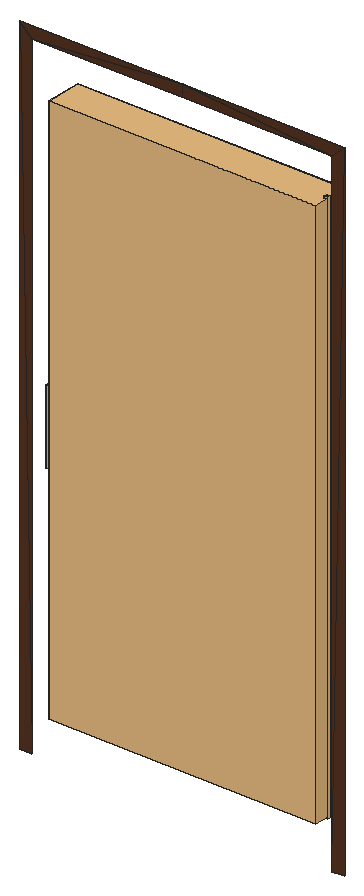
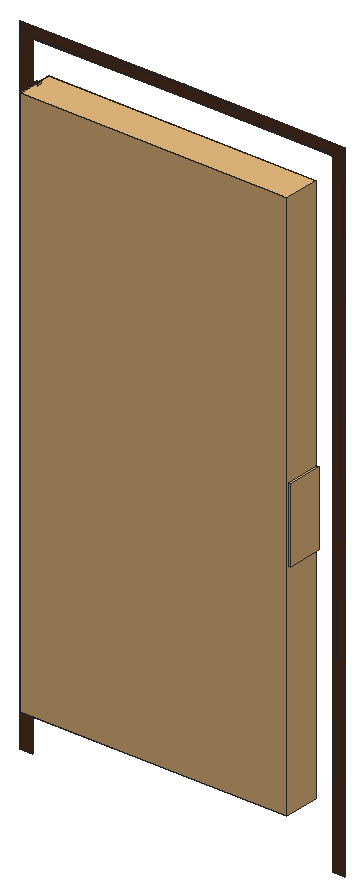
# SketchUp Ruby script. Lengths in inches.
U = 1.inch
M = Sketchup.active_model
def pt(a) = Geom::Point3d.new(a.map { |v| v * U })
def face(e, loops, mat)
  f = e.add_face(loops[0].map { |a| pt(a) })
  loops[1..].each { |l| e.add_face(l.map { |a| pt(a) }).erase! }
  f.material = f.back_material = mat if mat
  f
end
# faces: each face lists its corners as indices into pts; further lists are holes
def faces(e, pts, list, mat = nil) = list.each { |f| face(e, (f[0].is_a?(Array) ? f : [f]).map { |l| l.map { |i| pts[i] } }, mat) }
# xy, xz, yz: faces in a plane at the given z, y or x. An outline is a flat list of corners, or four numbers for a rectangle; further outlines are holes
def ring(l) = l.size == 4 ? [[l[0], l[1]], [l[2], l[1]], [l[2], l[3]], [l[0], l[3]]] : l.each_slice(2).to_a
def flat(e, list, mat, &to3) = list.each { |f| face(e, (f[0].is_a?(Array) ? f : [f]).map { |l| ring(l).map { |u, v| to3.(u, v) } }, mat) }
def xy(e, z, list, mat = nil) = flat(e, list, mat) { |x, y| [x, y, z] }
def xz(e, y, list, mat = nil) = flat(e, list, mat) { |x, z| [x, y, z] }
def yz(e, x, list, mat = nil) = flat(e, list, mat) { |y, z| [x, y, z] }
def lines(e, pts, list) = list.each { |a, b| e.add_line(pt(pts[a]), pt(pts[b])) }
# prism: a flat outline (further loops are holes) pulled along v
def prism(e, loops, v, mat = nil)
  f = face(e, loops, mat); d = Geom::Vector3d.new(v.map { |x| x * U })
  f.pushpull(f.normal.samedirection?(d) ? d.length : -d.length)
end
def box(e, o, s, mat = nil) = prism(e, [[o, [o[0] + s[0], o[1], o[2]], [o[0] + s[0], o[1] + s[1], o[2]], [o[0], o[1] + s[1], o[2]]]], [0, 0, s[2]], mat)
def at(x, y, z, deg = 0) = Geom::Transformation.translation(pt([x, y, z])) * Geom::Transformation.rotation(ORIGIN, Z_AXIS, deg.degrees)
def axes(o, x, y, z) = Geom::Transformation.new([*x, 0, *y, 0, *z, 0, *pt(o).to_a, 1])
def part(name) = M.definitions.add(name)
# library, detail: a bought-in or finely detailed component or shape, given as its bounding box
def library(name, o, s) = part(name).tap { |d| box(d.entities, o, s) }
def detail(e, o, s) = box(e.add_group.entities, o, s)
def put(e, d, t, mat = nil) = e.add_instance(d, t).tap { |i| i.material = mat if mat }
def group(e, t, mat = nil) = e.add_group.tap { |g| g.transformation = t; g.material = mat if mat }.entities
root = M.entities
M.materials.add("Material \#0").color = [86, 53, 35]
M.materials.add("Material \#1").color = [140, 140, 140]
c1 = library("3DGeom~7_Defintion",[455.56,-471.94,-18.85],[5.55,1000,5.48])
c2 = part("3DGeom~8_Defintion")
xz(c2.entities,-471.94,[[458.125,-17.29,459.53,-16.11,457.73,-17.15],[458.125,-17.29,458.54,-17.29,459.53,-16.11],[458.54,-17.29,458.93,-17.15,459.53,-16.11],[457.73,-17.15,459.53,-16.11,457.42,-16.88],[458.93,-17.15,459.25,-16.88,459.53,-16.11],
  [457.42,-16.88,459.53,-16.11,457.21,-16.52],[459.25,-16.88,459.46,-16.52,459.53,-16.11],[457.21,-16.52,459.53,-16.11,457.14,-16.11],[457.14,-16.11,459.53,-16.11,457.21,-15.7],[459.53,-16.11,457.42,-15.34,457.21,-15.7],
  [459.53,-16.11,457.73,-15.07,457.42,-15.34],[459.53,-16.11,458.125,-14.93,457.73,-15.07],[459.53,-16.11,458.54,-14.93,458.125,-14.93],[459.53,-16.11,458.93,-15.07,458.54,-14.93],[459.53,-16.11,459.25,-15.34,458.93,-15.07],
  [459.53,-16.11,459.46,-15.7,459.25,-15.34]],"Material \#1")
xz(c2.entities,-416.39,[[458.125,-17.29,457.73,-17.15,459.53,-16.11],[458.125,-17.29,459.53,-16.11,458.54,-17.29],[458.54,-17.29,459.53,-16.11,458.93,-17.15],[457.73,-17.15,457.42,-16.88,459.53,-16.11],[458.93,-17.15,459.53,-16.11,459.25,-16.88],
  [457.42,-16.88,457.21,-16.52,459.53,-16.11],[459.25,-16.88,459.53,-16.11,459.46,-16.52],[457.21,-16.52,457.14,-16.11,459.53,-16.11],[457.14,-16.11,457.21,-15.7,459.53,-16.11],[459.53,-16.11,457.21,-15.7,457.42,-15.34],
  [459.53,-16.11,457.42,-15.34,457.73,-15.07],[459.53,-16.11,457.73,-15.07,458.125,-14.93],[459.53,-16.11,458.125,-14.93,458.54,-14.93],[459.53,-16.11,458.54,-14.93,458.93,-15.07],[459.53,-16.11,458.93,-15.07,459.25,-15.34],
  [459.53,-16.11,459.25,-15.34,459.46,-15.7]],"Material \#1")
xz(c2.entities,-27.5,[[458.125,-17.29,459.53,-16.11,457.73,-17.15],[458.125,-17.29,458.54,-17.29,459.53,-16.11],[458.54,-17.29,458.93,-17.15,459.53,-16.11],[457.73,-17.15,459.53,-16.11,457.42,-16.88],[458.93,-17.15,459.25,-16.88,459.53,-16.11],
  [457.42,-16.88,459.53,-16.11,457.21,-16.52],[459.25,-16.88,459.46,-16.52,459.53,-16.11],[457.21,-16.52,459.53,-16.11,457.14,-16.11],[457.14,-16.11,459.53,-16.11,457.21,-15.7],[459.53,-16.11,457.42,-15.34,457.21,-15.7],
  [459.53,-16.11,457.73,-15.07,457.42,-15.34],[459.53,-16.11,458.125,-14.93,457.73,-15.07],[459.53,-16.11,458.54,-14.93,458.125,-14.93],[459.53,-16.11,458.93,-15.07,458.54,-14.93],[459.53,-16.11,459.25,-15.34,458.93,-15.07],
  [459.53,-16.11,459.46,-15.7,459.25,-15.34]],"Material \#1")
xz(c2.entities,28.06,[[458.125,-17.29,457.73,-17.15,459.53,-16.11],[458.125,-17.29,459.53,-16.11,458.54,-17.29],[458.54,-17.29,459.53,-16.11,458.93,-17.15],[457.73,-17.15,457.42,-16.88,459.53,-16.11],[458.93,-17.15,459.53,-16.11,459.25,-16.88],
  [457.42,-16.88,457.21,-16.52,459.53,-16.11],[459.25,-16.88,459.53,-16.11,459.46,-16.52],[457.21,-16.52,457.14,-16.11,459.53,-16.11],[457.14,-16.11,457.21,-15.7,459.53,-16.11],[459.53,-16.11,457.21,-15.7,457.42,-15.34],
  [459.53,-16.11,457.42,-15.34,457.73,-15.07],[459.53,-16.11,457.73,-15.07,458.125,-14.93],[459.53,-16.11,458.125,-14.93,458.54,-14.93],[459.53,-16.11,458.54,-14.93,458.93,-15.07],[459.53,-16.11,458.93,-15.07,459.25,-15.34],
  [459.53,-16.11,459.25,-15.34,459.46,-15.7]],"Material \#1")
xz(c2.entities,472.5,[[458.125,-17.29,459.53,-16.11,457.73,-17.15],[458.125,-17.29,458.54,-17.29,459.53,-16.11],[458.54,-17.29,458.93,-17.15,459.53,-16.11],[457.73,-17.15,459.53,-16.11,457.42,-16.88],[458.93,-17.15,459.25,-16.88,459.53,-16.11],
  [457.42,-16.88,459.53,-16.11,457.21,-16.52],[459.25,-16.88,459.46,-16.52,459.53,-16.11],[457.21,-16.52,459.53,-16.11,457.14,-16.11],[457.14,-16.11,459.53,-16.11,457.21,-15.7],[459.53,-16.11,457.42,-15.34,457.21,-15.7],
  [459.53,-16.11,457.73,-15.07,457.42,-15.34],[459.53,-16.11,458.125,-14.93,457.73,-15.07],[459.53,-16.11,458.54,-14.93,458.125,-14.93],[459.53,-16.11,458.93,-15.07,458.54,-14.93],[459.53,-16.11,459.25,-15.34,458.93,-15.07],
  [459.53,-16.11,459.46,-15.7,459.25,-15.34]],"Material \#1")
xz(c2.entities,528.06,[[458.125,-17.29,457.73,-17.15,459.53,-16.11],[458.125,-17.29,459.53,-16.11,458.54,-17.29],[458.54,-17.29,459.53,-16.11,458.93,-17.15],[457.73,-17.15,457.42,-16.88,459.53,-16.11],[458.93,-17.15,459.53,-16.11,459.25,-16.88],
  [457.42,-16.88,457.21,-16.52,459.53,-16.11],[459.25,-16.88,459.53,-16.11,459.46,-16.52],[457.21,-16.52,457.14,-16.11,459.53,-16.11],[457.14,-16.11,457.21,-15.7,459.53,-16.11],[459.53,-16.11,457.21,-15.7,457.42,-15.34],
  [459.53,-16.11,457.42,-15.34,457.73,-15.07],[459.53,-16.11,457.73,-15.07,458.125,-14.93],[459.53,-16.11,458.125,-14.93,458.54,-14.93],[459.53,-16.11,458.54,-14.93,458.93,-15.07],[459.53,-16.11,458.93,-15.07,459.25,-15.34],
  [459.53,-16.11,459.25,-15.34,459.46,-15.7]],"Material \#1")
c3 = part("3DGeom~21_Defintion")
xy(c3.entities,73.08,[[-976.3,-241.71,23.7,-241.71,-976.3,-223.46],[23.7,-241.71,5.45,-223.46,-976.3,-223.46],[23.7,-241.71,23.7,0,5.45,-223.46],[5.45,-223.46,23.7,0,5.45,0],[23.7,0,23.7,241.71,5.45,223.46],
  [5.45,0,23.7,0,5.45,223.46],[-976.3,223.46,23.7,241.71,-976.3,241.71],[-976.3,223.46,5.45,223.46,23.7,241.71]],"Material \#0")
c4 = library("3DGeom~6_Defintion",[-5.59,-471.8,-48.03],[468.87,1000,73.72])
c5 = library("3DGeom~3_Defintion",[-83.33,-500,-350],[620.1,1000,533.33])
xy(root,158.6113,[[371.5299,115.1498,371.4637,115.1703,371.4738,115.1852],[371.5299,115.1498,371.4738,115.1852,371.5335,115.1668],[371.5299,115.1498,371.5335,115.1668,371.6005,115.1498],[371.6005,115.1498,371.5335,115.1668,371.5969,115.1668],[371.6005,115.1498,371.5969,115.1668,371.6667,115.1703],
  [371.5969,115.1668,371.6566,115.1852,371.6667,115.1703],[371.4637,115.1703,371.4096,115.2088,371.4252,115.2199],[371.4637,115.1703,371.4252,115.2199,371.4738,115.1852],[371.6667,115.1703,371.6566,115.1852,371.7208,115.2088],[371.6566,115.1852,371.7052,115.2199,371.7208,115.2088],
  [371.4096,115.2088,371.3744,115.2607,371.3934,115.2666],[371.4096,115.2088,371.3934,115.2666,371.4252,115.2199],[371.7208,115.2088,371.7052,115.2199,371.756,115.2607],[371.7052,115.2199,371.737,115.2666,371.756,115.2607],[371.3744,115.2607,371.3621,115.3197,371.3824,115.3197],
  [371.3744,115.2607,371.3824,115.3197,371.3934,115.2666],[371.756,115.2607,371.737,115.2666,371.7683,115.3197],[371.737,115.2666,371.748,115.3197,371.7683,115.3197],[371.3621,115.3197,371.3744,115.3787,371.3934,115.3728],[371.3621,115.3197,371.3934,115.3728,371.3824,115.3197],
  [371.748,115.3197,371.737,115.3728,371.756,115.3787],[371.748,115.3197,371.756,115.3787,371.7683,115.3197],[371.3934,115.3728,371.3744,115.3787,371.4252,115.4195],[371.737,115.3728,371.7052,115.4195,371.7208,115.4306],[371.737,115.3728,371.7208,115.4306,371.756,115.3787],
  [371.3744,115.3787,371.4096,115.4306,371.4252,115.4195],[371.4252,115.4195,371.4096,115.4306,371.4738,115.4542],[371.7052,115.4195,371.6566,115.4542,371.6667,115.4691],[371.7052,115.4195,371.6667,115.4691,371.7208,115.4306],[371.4096,115.4306,371.4637,115.4691,371.4738,115.4542],
  [371.4738,115.4542,371.4637,115.4691,371.5335,115.4726],[371.6566,115.4542,371.5969,115.4726,371.6005,115.4896],[371.6566,115.4542,371.6005,115.4896,371.6667,115.4691],[371.4637,115.4691,371.5299,115.4896,371.5335,115.4726],[371.5335,115.4726,371.5299,115.4896,371.5969,115.4726],
  [371.5969,115.4726,371.5299,115.4896,371.6005,115.4896]],"Material \#1")
xy(root,158.6271,[[371.5299,115.1498,371.5335,115.1668,371.4637,115.1703],[371.5299,115.1498,371.5969,115.1668,371.5335,115.1668],[371.5299,115.1498,371.6005,115.1498,371.5969,115.1668],[371.6005,115.1498,371.6566,115.1852,371.5969,115.1668],[371.6005,115.1498,371.6667,115.1703,371.6566,115.1852],
  [371.5335,115.1668,371.4738,115.1852,371.4637,115.1703],[371.4637,115.1703,371.4738,115.1852,371.4096,115.2088],[371.6667,115.1703,371.7052,115.2199,371.6566,115.1852],[371.6667,115.1703,371.7208,115.2088,371.7052,115.2199],[371.4738,115.1852,371.4252,115.2199,371.4096,115.2088],
  [371.4096,115.2088,371.4252,115.2199,371.3744,115.2607],[371.7208,115.2088,371.737,115.2666,371.7052,115.2199],[371.7208,115.2088,371.756,115.2607,371.737,115.2666],[371.4252,115.2199,371.3934,115.2666,371.3744,115.2607],[371.3744,115.2607,371.3934,115.2666,371.3621,115.3197],
  [371.756,115.2607,371.748,115.3197,371.737,115.2666],[371.756,115.2607,371.7683,115.3197,371.748,115.3197],[371.3934,115.2666,371.3824,115.3197,371.3621,115.3197],[371.3621,115.3197,371.3824,115.3197,371.3744,115.3787],[371.3824,115.3197,371.3934,115.3728,371.3744,115.3787],
  [371.748,115.3197,371.7683,115.3197,371.737,115.3728],[371.7683,115.3197,371.756,115.3787,371.737,115.3728],[371.3934,115.3728,371.4096,115.4306,371.3744,115.3787],[371.3934,115.3728,371.4252,115.4195,371.4096,115.4306],[371.737,115.3728,371.756,115.3787,371.7052,115.4195],
  [371.756,115.3787,371.7208,115.4306,371.7052,115.4195],[371.4252,115.4195,371.4637,115.4691,371.4096,115.4306],[371.4252,115.4195,371.4738,115.4542,371.4637,115.4691],[371.7052,115.4195,371.7208,115.4306,371.6566,115.4542],[371.7208,115.4306,371.6667,115.4691,371.6566,115.4542],
  [371.4738,115.4542,371.5299,115.4896,371.4637,115.4691],[371.4738,115.4542,371.5335,115.4726,371.5299,115.4896],[371.6566,115.4542,371.6667,115.4691,371.5969,115.4726],[371.6667,115.4691,371.6005,115.4896,371.5969,115.4726],[371.5335,115.4726,371.6005,115.4896,371.5299,115.4896],
  [371.5335,115.4726,371.5969,115.4726,371.6005,115.4896]],"Material \#1")
xy(root,162.1701,[[371.5299,115.1498,371.4637,115.1703,371.5335,115.1668],[371.5299,115.1498,371.5335,115.1668,371.5969,115.1668],[371.5299,115.1498,371.5969,115.1668,371.6005,115.1498],[371.6005,115.1498,371.5969,115.1668,371.6566,115.1852],[371.6005,115.1498,371.6566,115.1852,371.6667,115.1703],
  [371.5335,115.1668,371.4637,115.1703,371.4738,115.1852],[371.4637,115.1703,371.4096,115.2088,371.4738,115.1852],[371.6667,115.1703,371.6566,115.1852,371.7052,115.2199],[371.6667,115.1703,371.7052,115.2199,371.7208,115.2088],[371.4738,115.1852,371.4096,115.2088,371.4252,115.2199],
  [371.4096,115.2088,371.3744,115.2607,371.4252,115.2199],[371.7208,115.2088,371.7052,115.2199,371.737,115.2666],[371.7208,115.2088,371.737,115.2666,371.756,115.2607],[371.4252,115.2199,371.3744,115.2607,371.3934,115.2666],[371.3744,115.2607,371.3621,115.3197,371.3934,115.2666],
  [371.756,115.2607,371.737,115.2666,371.748,115.3197],[371.756,115.2607,371.748,115.3197,371.7683,115.3197],[371.3934,115.2666,371.3621,115.3197,371.3824,115.3197],[371.3621,115.3197,371.3744,115.3787,371.3824,115.3197],[371.3824,115.3197,371.3744,115.3787,371.3934,115.3728],
  [371.748,115.3197,371.737,115.3728,371.7683,115.3197],[371.7683,115.3197,371.737,115.3728,371.756,115.3787],[371.3934,115.3728,371.3744,115.3787,371.4096,115.4306],[371.3934,115.3728,371.4096,115.4306,371.4252,115.4195],[371.737,115.3728,371.7052,115.4195,371.756,115.3787],
  [371.756,115.3787,371.7052,115.4195,371.7208,115.4306],[371.4252,115.4195,371.4096,115.4306,371.4637,115.4691],[371.4252,115.4195,371.4637,115.4691,371.4738,115.4542],[371.7052,115.4195,371.6566,115.4542,371.7208,115.4306],[371.7208,115.4306,371.6566,115.4542,371.6667,115.4691],
  [371.4738,115.4542,371.4637,115.4691,371.5299,115.4896],[371.4738,115.4542,371.5299,115.4896,371.5335,115.4726],[371.6566,115.4542,371.5969,115.4726,371.6667,115.4691],[371.6667,115.4691,371.5969,115.4726,371.6005,115.4896],[371.5335,115.4726,371.5299,115.4896,371.6005,115.4896],
  [371.5335,115.4726,371.6005,115.4896,371.5969,115.4726]],"Material \#1")
xy(root,162.1859,[[371.5299,115.1498,371.4738,115.1852,371.4637,115.1703],[371.5299,115.1498,371.5335,115.1668,371.4738,115.1852],[371.5299,115.1498,371.6005,115.1498,371.5335,115.1668],[371.6005,115.1498,371.5969,115.1668,371.5335,115.1668],[371.6005,115.1498,371.6667,115.1703,371.5969,115.1668],
  [371.5969,115.1668,371.6667,115.1703,371.6566,115.1852],[371.4637,115.1703,371.4252,115.2199,371.4096,115.2088],[371.4637,115.1703,371.4738,115.1852,371.4252,115.2199],[371.6667,115.1703,371.7208,115.2088,371.6566,115.1852],[371.6566,115.1852,371.7208,115.2088,371.7052,115.2199],
  [371.4096,115.2088,371.3934,115.2666,371.3744,115.2607],[371.4096,115.2088,371.4252,115.2199,371.3934,115.2666],[371.7208,115.2088,371.756,115.2607,371.7052,115.2199],[371.7052,115.2199,371.756,115.2607,371.737,115.2666],[371.3744,115.2607,371.3824,115.3197,371.3621,115.3197],
  [371.3744,115.2607,371.3934,115.2666,371.3824,115.3197],[371.756,115.2607,371.7683,115.3197,371.737,115.2666],[371.737,115.2666,371.7683,115.3197,371.748,115.3197],[371.3621,115.3197,371.3824,115.3197,371.3934,115.3728],[371.3621,115.3197,371.3934,115.3728,371.3744,115.3787],
  [371.748,115.3197,371.756,115.3787,371.737,115.3728],[371.748,115.3197,371.7683,115.3197,371.756,115.3787],[371.3934,115.3728,371.4252,115.4195,371.3744,115.3787],[371.737,115.3728,371.7208,115.4306,371.7052,115.4195],[371.737,115.3728,371.756,115.3787,371.7208,115.4306],
  [371.3744,115.3787,371.4252,115.4195,371.4096,115.4306],[371.4252,115.4195,371.4738,115.4542,371.4096,115.4306],[371.7052,115.4195,371.6667,115.4691,371.6566,115.4542],[371.7052,115.4195,371.7208,115.4306,371.6667,115.4691],[371.4096,115.4306,371.4738,115.4542,371.4637,115.4691],
  [371.4738,115.4542,371.5335,115.4726,371.4637,115.4691],[371.6566,115.4542,371.6005,115.4896,371.5969,115.4726],[371.6566,115.4542,371.6667,115.4691,371.6005,115.4896],[371.4637,115.4691,371.5335,115.4726,371.5299,115.4896],[371.5335,115.4726,371.5969,115.4726,371.5299,115.4896],
  [371.5969,115.4726,371.6005,115.4896,371.5299,115.4896]],"Material \#1")
xy(root,190.2095,[[371.5299,115.1498,371.4637,115.1703,371.4738,115.1852],[371.5299,115.1498,371.4738,115.1852,371.5335,115.1668],[371.5299,115.1498,371.5335,115.1668,371.6005,115.1498],[371.6005,115.1498,371.5335,115.1668,371.5969,115.1668],[371.6005,115.1498,371.5969,115.1668,371.6667,115.1703],
  [371.5969,115.1668,371.6566,115.1852,371.6667,115.1703],[371.4637,115.1703,371.4096,115.2088,371.4252,115.2199],[371.4637,115.1703,371.4252,115.2199,371.4738,115.1852],[371.6667,115.1703,371.6566,115.1852,371.7208,115.2088],[371.6566,115.1852,371.7052,115.2199,371.7208,115.2088],
  [371.4096,115.2088,371.3744,115.2607,371.3934,115.2666],[371.4096,115.2088,371.3934,115.2666,371.4252,115.2199],[371.7208,115.2088,371.7052,115.2199,371.756,115.2607],[371.7052,115.2199,371.737,115.2666,371.756,115.2607],[371.3744,115.2607,371.3621,115.3197,371.3824,115.3197],
  [371.3744,115.2607,371.3824,115.3197,371.3934,115.2666],[371.756,115.2607,371.737,115.2666,371.7683,115.3197],[371.737,115.2666,371.748,115.3197,371.7683,115.3197],[371.3621,115.3197,371.3744,115.3787,371.3934,115.3728],[371.3621,115.3197,371.3934,115.3728,371.3824,115.3197],
  [371.748,115.3197,371.737,115.3728,371.756,115.3787],[371.748,115.3197,371.756,115.3787,371.7683,115.3197],[371.3934,115.3728,371.3744,115.3787,371.4252,115.4195],[371.737,115.3728,371.7052,115.4195,371.7208,115.4306],[371.737,115.3728,371.7208,115.4306,371.756,115.3787],
  [371.3744,115.3787,371.4096,115.4306,371.4252,115.4195],[371.4252,115.4195,371.4096,115.4306,371.4738,115.4542],[371.7052,115.4195,371.6566,115.4542,371.6667,115.4691],[371.7052,115.4195,371.6667,115.4691,371.7208,115.4306],[371.4096,115.4306,371.4637,115.4691,371.4738,115.4542],
  [371.4738,115.4542,371.4637,115.4691,371.5335,115.4726],[371.6566,115.4542,371.5969,115.4726,371.6005,115.4896],[371.6566,115.4542,371.6005,115.4896,371.6667,115.4691],[371.4637,115.4691,371.5299,115.4896,371.5335,115.4726],[371.5335,115.4726,371.5299,115.4896,371.5969,115.4726],
  [371.5969,115.4726,371.5299,115.4896,371.6005,115.4896]],"Material \#1")
xy(root,190.2253,[[371.5299,115.1498,371.5335,115.1668,371.4637,115.1703],[371.5299,115.1498,371.5969,115.1668,371.5335,115.1668],[371.5299,115.1498,371.6005,115.1498,371.5969,115.1668],[371.6005,115.1498,371.6566,115.1852,371.5969,115.1668],[371.6005,115.1498,371.6667,115.1703,371.6566,115.1852],
  [371.5335,115.1668,371.4738,115.1852,371.4637,115.1703],[371.4637,115.1703,371.4738,115.1852,371.4096,115.2088],[371.6667,115.1703,371.7052,115.2199,371.6566,115.1852],[371.6667,115.1703,371.7208,115.2088,371.7052,115.2199],[371.4738,115.1852,371.4252,115.2199,371.4096,115.2088],
  [371.4096,115.2088,371.4252,115.2199,371.3744,115.2607],[371.7208,115.2088,371.737,115.2666,371.7052,115.2199],[371.7208,115.2088,371.756,115.2607,371.737,115.2666],[371.4252,115.2199,371.3934,115.2666,371.3744,115.2607],[371.3744,115.2607,371.3934,115.2666,371.3621,115.3197],
  [371.756,115.2607,371.748,115.3197,371.737,115.2666],[371.756,115.2607,371.7683,115.3197,371.748,115.3197],[371.3934,115.2666,371.3824,115.3197,371.3621,115.3197],[371.3621,115.3197,371.3824,115.3197,371.3744,115.3787],[371.3824,115.3197,371.3934,115.3728,371.3744,115.3787],
  [371.748,115.3197,371.7683,115.3197,371.737,115.3728],[371.7683,115.3197,371.756,115.3787,371.737,115.3728],[371.3934,115.3728,371.4096,115.4306,371.3744,115.3787],[371.3934,115.3728,371.4252,115.4195,371.4096,115.4306],[371.737,115.3728,371.756,115.3787,371.7052,115.4195],
  [371.756,115.3787,371.7208,115.4306,371.7052,115.4195],[371.4252,115.4195,371.4637,115.4691,371.4096,115.4306],[371.4252,115.4195,371.4738,115.4542,371.4637,115.4691],[371.7052,115.4195,371.7208,115.4306,371.6566,115.4542],[371.7208,115.4306,371.6667,115.4691,371.6566,115.4542],
  [371.4738,115.4542,371.5299,115.4896,371.4637,115.4691],[371.4738,115.4542,371.5335,115.4726,371.5299,115.4896],[371.6566,115.4542,371.6667,115.4691,371.5969,115.4726],[371.6667,115.4691,371.6005,115.4896,371.5969,115.4726],[371.5335,115.4726,371.6005,115.4896,371.5299,115.4896],
  [371.5335,115.4726,371.5969,115.4726,371.6005,115.4896]],"Material \#1")
xy(root,190.5551,[[338.0267,116.355,338.0855,116.355,338.0855,116.6759]],"Material \#1")
xz(root,116.3205,[[338.0558,189.7138,338.1237,189.729,338.0912,189.7177],[337.988,189.729,338.2061,189.8295,338.1237,189.729],[338.1237,189.729,338.1763,189.77,338.1523,189.7468],[338.1237,189.729,338.2061,189.8295,338.1763,189.77],[338.1763,189.77,338.2061,189.8295,338.1945,189.7979],
  [338.2061,189.8295,337.8956,190.1739,338.2102,189.8639],[338.2102,189.8639,338,190.1664,338.0558,190.1601],[338.2102,189.8639,338.0558,190.1601,338.1117,190.1664],[338.2102,189.8639,338.1117,190.1664,338.2102,190.151],[338.2102,190.151,338.1117,190.1664,338.2118,190.1636],
  [338.2102,190.151,338.2118,190.1636,338.2106,190.1576],[338.2118,190.1636,338.1117,190.1664,338.2165,190.1744],[338.2118,190.1636,338.2165,190.1744,338.2137,190.1692],[338.1117,190.1664,338.163,190.1842,338.2165,190.1744],[338.2165,190.1744,338.163,190.1842,338.2082,190.2122],
  [338.2165,190.1744,338.2082,190.2122,338.246,190.2489],[338.2165,190.1744,338.246,190.2489,338.3295,190.3617],[338.2165,190.1744,338.3295,190.3617,338.2199,190.1792],[338.2199,190.1792,338.3295,190.3617,338.2241,190.1839],[338.2241,190.1839,338.2761,190.2374,338.229,190.1883],
  [338.2241,190.1839,338.3295,190.3617,338.2761,190.2374],[338.229,190.1883,338.2761,190.2374,338.2539,190.2116],[338.2761,190.2374,338.3107,190.2957,338.2952,190.2655],[338.2761,190.2374,338.3295,190.3617,338.3107,190.2957],[338.246,190.2489,338.2748,190.2929,338.3295,190.3617],
  [338.2748,190.2929,338.2931,190.3428,338.3295,190.3617],[338.3107,190.2957,338.3295,190.3617,338.3223,190.3278],[338.2931,190.3428,338.2995,190.3971,338.3295,190.3617],[338.3295,190.3617,338.2713,190.565,338.3247,190.4586],[338.3295,190.3617,338.2931,190.4514,338.2713,190.565],
  [338.3295,190.3617,338.2995,190.3971,338.2931,190.4514],[338.3295,190.3617,338.3247,190.4586,338.332,190.3971],[338.2931,190.4514,338.2748,190.5012,338.2713,190.565],[338.3247,190.4586,338.2713,190.565,338.3039,190.5151],[338.2748,190.5012,338.246,190.5453,338.2713,190.565],
  [338.246,190.5453,338.2082,190.582,338.2713,190.565],[338.2713,190.565,338.0558,190.6657,338.1772,190.6383],[338.2713,190.565,338.163,190.61,338.0558,190.6657],[338.2713,190.565,338.2082,190.582,338.163,190.61],[338.2713,190.565,338.1772,190.6383,338.2285,190.6066],
  [338.163,190.61,338.1117,190.6278,338.0558,190.6657],[338.1117,190.6278,338.0558,190.6341,338.0558,190.6657],[338.1772,190.6383,338.0558,190.6657,338.1191,190.6586]],"Material \#1")
xz(root,116.631,[[338.5991,187.5823,338.6587,187.6848,338.5897,187.59],[338.5991,187.5823,338.6692,187.6788,338.6587,187.6848],[338.2596,187.6349,338.2771,187.6707,338.2656,187.6749],[338.2771,187.6707,338.2761,187.7118,338.2656,187.6749],[338.2771,187.6707,338.2881,187.7097,338.2761,187.7118],
  [338.6692,187.6788,338.7103,187.7904,338.6587,187.6848],[338.6692,187.6788,338.7218,187.7863,338.7103,187.7904],[338.2919,187.7507,338.2881,187.7918,338.2761,187.7897],[338.7218,187.7863,338.7427,187.9051,338.7103,187.7904],[338.7218,187.7863,338.7548,187.903,338.7427,187.9051],
  [338.2761,187.7897,338.2881,187.7918,338.2656,187.8266],[338.2881,187.7918,338.2771,187.8308,338.2656,187.8266],[338.7548,187.903,338.7545,188.0322,338.7427,187.9051],[338.7548,187.903,338.7666,188.0316,338.7545,188.0322],[338.7666,188.0316,338.7545,194.2213,338.7545,188.0322],
  [338.7666,188.0316,338.7545,195.9218,338.7545,194.2213],[338.7666,188.0316,338.7666,195.9223,338.7545,195.9218]],"Material \#1")
yz(root,338.0796,[[116.355,190.326,116.6759,190.326,116.355,190.3536],[116.6759,190.326,116.6759,190.3536,116.355,190.3536]],"Material \#1")
yz(root,338.0855,[[116.355,190.4366,116.6759,190.4366,116.355,190.4879]],"Material \#1")
yz(root,338.0886,[[116.355,190.376,116.6759,190.376,116.355,190.3984],[116.6759,190.376,116.6759,190.3984,116.355,190.3984]],"Material \#1")
p = [[338.0679,116.355,190.2628],[338.0796,116.355,190.2391],[338.0796,116.6759,190.2391],[338.0796,116.6759,190.2391],[338.071,116.6759,190.2667],[338.0679,116.355,190.2628],
  [338.0796,116.355,190.326],[338.0679,116.355,190.2964],[338.071,116.6759,190.2924],[338.071,116.6759,190.2924],[338.0679,116.355,190.2964],[338.0741,116.355,190.2884],
  [338.071,116.6759,190.2667],[338.0741,116.355,190.2707],[338.0679,116.355,190.2628],[338.071,116.6759,190.2667],[338.071,116.6759,190.2924],[338.0741,116.355,190.2884],
  [338.0741,116.355,190.2707],[338.071,116.6759,190.2924],[338.0796,116.6759,190.326],[338.0796,116.355,190.326],[338.0796,116.355,190.4208],[338.0886,116.355,190.3984],
  [338.0886,116.6759,190.3984],[338.0855,116.355,190.4366],[338.0796,116.355,190.4208],[338.0796,116.6759,190.4208],[338.0796,116.6759,190.3536],[338.0886,116.6759,190.376],
  [338.0886,116.355,190.376],[338.0796,116.355,190.3536],[338.0886,116.6759,190.3984],[338.0796,116.6759,190.4208],[338.0796,116.355,190.4208],[338.0796,116.6759,190.4208],
  [338.0855,116.6759,190.4366],[338.0855,116.355,190.4366],[338.0855,116.6759,190.4366],[338.0824,116.6759,190.4975],[338.0855,116.355,190.4879],[338.0855,116.355,190.5551],
  [338.0855,116.355,190.5037],[338.0824,116.6759,190.4975],[338.0824,116.6759,190.4975],[338.0855,116.6759,190.5551],[338.0855,116.355,190.5551]]
faces(root,p,[[0,1,2],[3,4,5],[6,7,8],[9,10,11],[12,13,14],[15,16,17],[17,18,15],[19,20,21],
  [22,23,24],[25,26,27],[28,29,30],[30,31,28],[32,33,34],[35,36,37],[38,39,40],[41,42,43],
  [44,45,46]],"Material \#1")
put(root,c1,axes([338.06,116.32,191.98],[0.07311,0,0],[0,0,0.0711],[0,0.06212,0]),"Material \#1")
put(root,c2,axes([338.06,116.32,191.98],[0.07311,0,0],[0,0,0.0711],[0,0.06212,0]),"Material \#1")
put(root,c3,axes([353.08,120.67,233.84],[0,0,0.08334],[0.0857,0,0],[0,-0.07281,0]),"Material \#0")
put(root,c4,axes([338.06,116.32,191.98],[0.07273,0,0],[0,0,0.07072],[0,0.06179,0]),"Material \#1")
put(root,c5,axes([338.06,116.32,191.98],[0.00975,0,0],[0,0,0.00948],[0,0.00828,0]),"Material \#1")
